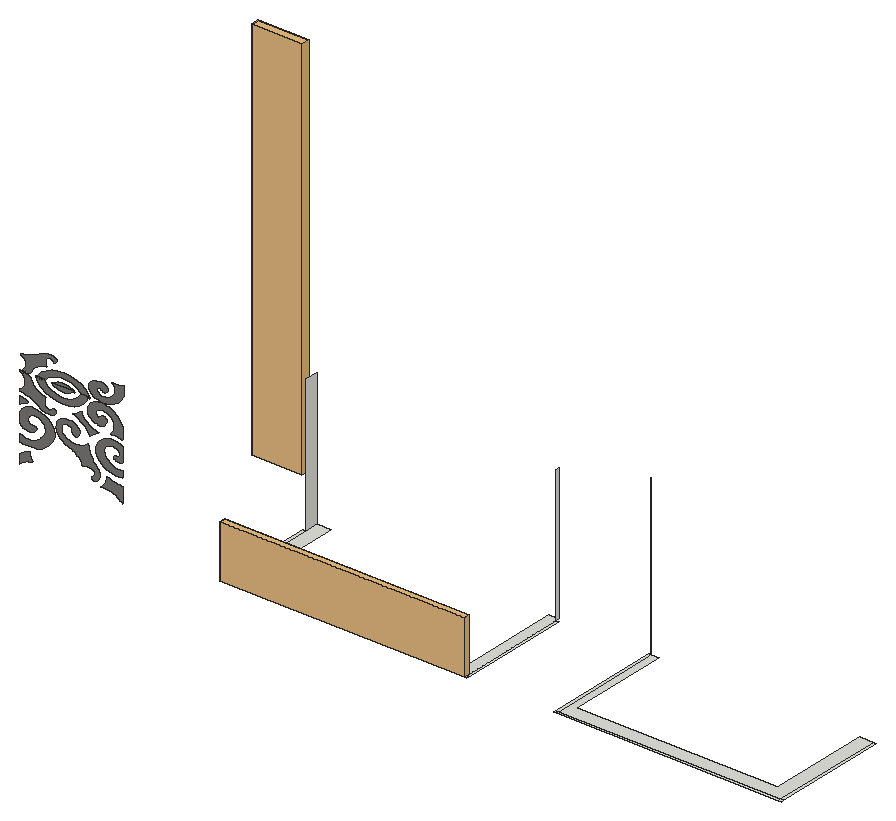
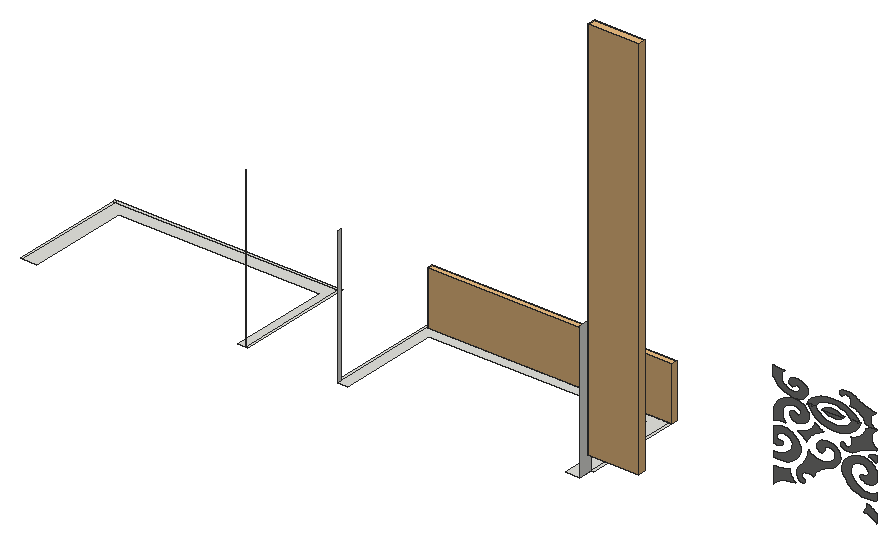
# SketchUp Ruby script. Lengths in inches.
U = 1.inch
M = Sketchup.active_model
def pt(a) = Geom::Point3d.new(a.map { |v| v * U })
def face(e, loops, mat)
  f = e.add_face(loops[0].map { |a| pt(a) })
  loops[1..].each { |l| e.add_face(l.map { |a| pt(a) }).erase! }
  f.material = f.back_material = mat if mat
  f
end
# faces: each face lists its corners as indices into pts; further lists are holes
def faces(e, pts, list, mat = nil) = list.each { |f| face(e, (f[0].is_a?(Array) ? f : [f]).map { |l| l.map { |i| pts[i] } }, mat) }
# xy, xz, yz: faces in a plane at the given z, y or x. An outline is a flat list of corners, or four numbers for a rectangle; further outlines are holes
def ring(l) = l.size == 4 ? [[l[0], l[1]], [l[2], l[1]], [l[2], l[3]], [l[0], l[3]]] : l.each_slice(2).to_a
def flat(e, list, mat, &to3) = list.each { |f| face(e, (f[0].is_a?(Array) ? f : [f]).map { |l| ring(l).map { |u, v| to3.(u, v) } }, mat) }
def xy(e, z, list, mat = nil) = flat(e, list, mat) { |x, y| [x, y, z] }
def xz(e, y, list, mat = nil) = flat(e, list, mat) { |x, z| [x, y, z] }
def yz(e, x, list, mat = nil) = flat(e, list, mat) { |y, z| [x, y, z] }
def lines(e, pts, list) = list.each { |a, b| e.add_line(pt(pts[a]), pt(pts[b])) }
# prism: a flat outline (further loops are holes) pulled along v
def prism(e, loops, v, mat = nil)
  f = face(e, loops, mat); d = Geom::Vector3d.new(v.map { |x| x * U })
  f.pushpull(f.normal.samedirection?(d) ? d.length : -d.length)
end
def box(e, o, s, mat = nil) = prism(e, [[o, [o[0] + s[0], o[1], o[2]], [o[0] + s[0], o[1] + s[1], o[2]], [o[0], o[1] + s[1], o[2]]]], [0, 0, s[2]], mat)
def at(x, y, z, deg = 0) = Geom::Transformation.translation(pt([x, y, z])) * Geom::Transformation.rotation(ORIGIN, Z_AXIS, deg.degrees)
def axes(o, x, y, z) = Geom::Transformation.new([*x, 0, *y, 0, *z, 0, *pt(o).to_a, 1])
def part(name) = M.definitions.add(name)
# library, detail: a bought-in or finely detailed component or shape, given as its bounding box
def library(name, o, s) = part(name).tap { |d| box(d.entities, o, s) }
def detail(e, o, s) = box(e.add_group.entities, o, s)
def put(e, d, t, mat = nil) = e.add_instance(d, t).tap { |i| i.material = mat if mat }
def group(e, t, mat = nil) = e.add_group.tap { |g| g.transformation = t; g.material = mat if mat }.entities
root = M.entities
M.materials.add("[0043_SaddleBrown]4").color = [124, 123, 122]
M.materials.add("[Granite Light Gray]").color = [149, 148, 144]
c1 = library("Scandinavian Door w/ Glass Wall\#2",[-41.94,78.85,0],[6.47,62.99,82.68])
c2 = library("Glass Railing",[0,0,0],[139.5,4.76,42])
xy(root,413.5,[[3051.26,557.9375,3243.69,559.875],[3243.69,557.9375,3245.63,559.875],[3314.21,557.9375,3316.14,559.875],[3316.14,557.9375,3491.44,559.875],[3491.44,557.9375,3493.37,559.875],
  [3051.07,559.875,3053.01,640.11],[3053.01,559.875,3243.69,559.875,3243.69,651.03,3235.84,651.03,3235.84,570.83,3064.33,570.83,3064.33,651.03,3053.01,651.03],[3243.69,559.875,3245.63,647.91],[3314.21,559.875,3316.14,651.03],[3316.14,559.875,3491.44,559.875,3491.44,651.03,3480.11,651.03,3480.11,570.83,3322.22,570.83,3322.22,651.03,3316.14,651.03],
  [3491.44,559.875,3493.37,651.03]])
xz(root,589.17,[[2949.62,418.4,2949.62,430.94,2948.58,430.96,2947.54,431.01,2946.51,431.09,2945.48,431.2,2944.46,431.34,2943.45,431.51,2942.44,431.7,2941.45,431.93,2940.47,432.18,2939.51,432.46,2938.5625,432.77,2937.63,433.11,2937.53,432.33,2937.37,431.56,2937.16,430.79,2936.89,430.03,2936.57,429.29,2936.2,428.55,2935.78,427.83,2935.3,427.13,2934.78,426.44,2934.21,425.78,2933.59,425.14,2932.93,424.52,2934.59,424.625,2936.25,424.61,2937.9,424.48,2939.52,424.22,2941.1,423.85,2942.61,423.36,2944.05,422.76,2945.4,422.0625,2946.64,421.27,2947.77,420.39,2948.76,419.43],[2869.23,418.5,2869.75,419.14,2870.34,419.74,2870.99,420.3125,2871.71,420.84,2872.49,421.32,2873.32,421.76,2874.19,422.14,2875.11,422.48,2876.06,422.75,2877.03,422.98,2878.03,423.14,2879.05,423.24,2878.63,423.73,2878.25,424.24,2877.9,424.76,2877.6,425.29,2877.33,425.83,2877.1,426.38,2876.91,426.94,2876.76,427.51,2876.65,428.08,2876.58,428.65,2876.55,429.23,2876.57,429.8,2875.87,429.54,2875.19,429.27,2874.51,428.97,2873.86,428.66,2873.22,428.33,2872.59,427.99,2871.98,427.63,2871.39,427.26,2870.82,426.87,2870.27,426.47,2869.74,426.05,2869.23,425.62],[2927.3,427.2,2927.86,427.23,2928.4,427.32,2928.93,427.46,2929.41,427.66,2929.86,427.9,2930.25,428.18,2930.58,428.51,2930.85,428.86,2931.04,429.24,2931.16,429.63,2931.19,430.04,2931.41,430.71,2931.55,431.38,2931.63,432.07,2931.64,432.76,2931.57,433.44,2931.44,434.125,2931.24,434.8,2930.98,435.46,2930.64,436.1,2930.24,436.72,2929.79,437.33,2929.27,437.9,2928.33,438.91,2927.46,439.95,2926.66,441.02,2925.92,442.11,2925.25,443.22,2924.66,444.36,2924.13,445.51,2923.68,446.68,2923.3,447.86,2923,449.05,2922.77,450.26,2922.62,451.46,2921.65,450.57,2920.53,449.77,2919.28,449.08,2917.91,448.52,2916.45,448.09,2914.93,447.8,2913.37,447.66,2911.79,447.66,2910.23,447.8125,2908.71,448.11,2907.26,448.54,2905.89,449.11,2904.92,449.65,2904.05,450.27,2903.3,450.97,2902.68,451.74,2902.2,452.55,2901.875,453.4,2901.7,454.28,2901.68,455.16,2901.82,456.04,2902.12,456.9,2902.57,457.72,2903.16,458.5,2903.7,458.79,2904.31,459.03,2904.95,459.19,2905.62,459.29,2906.3,459.31,2906.98,459.26,2907.64,459.13,2908.27,458.94,2908.85,458.68,2909.37,458.36,2909.82,457.99,2910.1875,457.57,2910.07,457.28,2909.98,456.98,2909.93,456.67,2909.91,456.37,2909.92,456.06,2909.97,455.75,2910.05,455.45,2910.16,455.16,2910.31,454.87,2910.49,454.59,2910.7,454.32,2910.93,454.0625,2911.16,453.87,2911.4375,453.7,2911.74,453.5625,2912.07,453.47,2912.42,453.41,2912.78,453.38,2913.14,453.41,2913.48,453.47,2913.82,453.5625,2914.12,453.7,2914.39,453.87,2914.625,454.0625,2915.3,454.87,2915.77,455.75,2916.03,456.67,2916.0625,457.61,2915.875,458.54,2915.47,459.4375,2914.85,460.27,2914.05,461.01,2913.09,461.64,2911.99,462.15,2910.78,462.51,2909.51,462.72,2908.09,462.91,2906.65,462.94,2905.21,462.8125,2903.83,462.53,2902.51,462.1,2901.3,461.53,2900.23,460.83,2899.32,460.03,2898.58,459.13,2898.04,458.17,2897.72,457.15,2897.61,456.12,2897.49,454.92,2897.56,453.72,2897.79,452.53,2898.19,451.37,2898.76,450.24,2899.49,449.16,2900.37,448.14,2901.39,447.19,2902.54,446.32,2903.81,445.55,2905.18,444.87,2906.65,444.3,2908.04,443.78,2909.37,443.1875,2910.64,442.53,2911.85,441.81,2912.98,441.03,2914.03,440.19,2914.99,439.31,2915.87,438.37,2916.65,437.39,2917.34,436.38,2917.92,435.33,2918.4,434.26,2919.08,434.625,2919.82,434.93,2920.61,435.15,2921.43,435.3,2922.28,435.36,2923.13,435.34,2923.97,435.24,2924.78,435.05,2925.55,434.79,2926.26,434.46,2926.9,434.06,2927.47,433.6,2927.67,433.23,2927.82,432.84,2927.9,432.45,2927.93,432.05,2927.89,431.65,2927.78,431.26,2927.62,430.875,2927.4,430.51,2927.125,430.16,2926.79,429.84,2926.42,429.55,2926,429.29,2925.77,429.13,2925.58,428.95,2925.45,428.75,2925.38,428.53,2925.37,428.3,2925.42,428.08,2925.53,427.87,2925.69,427.67,2925.9,427.51,2926.16,427.375,2926.44,427.28,2926.75,427.23],[2875.84,433.3,2878.1,433.36,2880.34,433.62,2882.51,434.07,2884.6,434.7,2886.5625,435.5,2888.38,436.47,2890.02,437.59,2891.47,438.85,2892.7,440.22,2894.37,442.26,2895.52,444.47,2896.14,446.8,2896.18,449.17,2895.66,451.51,2894.59,453.75,2893,455.82,2890.9375,457.67,2888.46,459.23,2885.66,460.46,2882.6,461.32,2879.38,461.79,2878.22,461.63,2877.08,461.4,2875.99,461.08,2874.9375,460.69,2873.94,460.24,2873.01,459.71,2872.16,459.125,2871.38,458.48,2870.7,457.79,2870.11,457.06,2869.61,456.28,2869.23,455.48,2869.23,447.4,2869.76,446.49,2870.53,445.68,2871.52,445,2872.68,444.48,2873.96,444.15,2875.3,444,2876.67,444.0625,2877.98,444.32,2879.2,444.76,2880.26,445.37,2881.13,446.13,2881.77,447,2881.87,447.21,2881.92,447.42,2881.92,447.64,2881.88,447.86,2881.8,448.07,2881.67,448.27,2881.51,448.46,2881.31,448.62,2881.07,448.76,2880.82,448.88,2880.54,448.97,2880.24,449.02,2879.51,448.93,2878.78,448.94,2878.06,449.05,2877.375,449.25,2876.75,449.54,2876.22,449.9,2875.78,450.33,2875.47,450.81,2875.28,451.32,2875.22,451.85,2875.31,452.38,2875.52,452.89,2875.7,453.55,2876.03,454.18,2876.49,454.77,2877.07,455.29,2877.76,455.75,2878.53,456.12,2879.38,456.4,2880.28,456.57,2881.21,456.65,2882.14,456.62,2883.06,456.48,2883.93,456.24,2885.28,455.45,2886.47,454.53,2887.47,453.51,2888.25,452.39,2888.8125,451.2,2889.13,449.96,2889.2,448.71,2889.03,447.46,2888.61,446.24,2887.96,445.08,2887.09,443.99,2886.01,443.01,2885.57,442.35,2885.06,441.73,2884.47,441.14,2883.83,440.59,2883.12,440.07,2882.35,439.6,2881.53,439.18,2880.67,438.8125,2879.76,438.49,2878.82,438.23,2877.86,438.03,2876.875,437.88,2876.17,437.82,2875.47,437.8,2874.76,437.83,2874.0625,437.89,2873.37,438,2872.7,438.16,2872.04,438.35,2871.41,438.58,2870.8125,438.85,2870.24,439.15,2869.71,439.48,2869.23,439.85,2869.23,434.28,2871.37,433.76,2873.59,433.44],[2947.02,436.71,2949.62,436.96,2949.62,441.66,2947.39,441.61,2945.18,441.84,2943.06,442.34,2941.09,443.09,2939.33,444.09,2937.84,445.28,2936.66,446.65,2935.83,448.14,2935.37,449.72,2935.3,451.32,2935.62,452.92,2936.3125,454.45,2937.11,455.1,2938.06,455.63,2939.13,456.03,2940.29,456.27,2941.49,456.35,2942.7,456.27,2943.85,456.02,2944.93,455.625,2945.875,455.09,2946.67,454.43,2947.28,453.68,2947.68,452.86,2947.75,452.53,2947.74,452.1875,2947.66,451.86,2947.49,451.54,2947.25,451.25,2946.95,450.99,2946.59,450.77,2946.1875,450.61,2945.75,450.49,2945.29,450.43,2944.82,450.42,2944.36,450.48,2944.12,450.4,2943.89,450.31,2943.68,450.19,2943.48,450.06,2943.31,449.92,2943.15,449.77,2943.03,449.6,2942.92,449.42,2942.85,449.24,2942.8,449.06,2942.78,448.87,2942.79,448.68,2943.15,448.29,2943.59,447.9375,2944.09,447.63,2944.64,447.38,2945.23,447.18,2945.85,447.04,2946.49,446.96,2947.14,446.9375,2947.79,446.98,2948.43,447.09,2949.04,447.25,2949.62,447.47,2949.62,459.11,2948.55,459.72,2947.4,460.23,2946.16,460.64,2944.87,460.9375,2943.53,461.12,2942.18,461.18,2940.82,461.12,2939.48,460.9375,2938.1875,460.64,2936.95,460.23,2935.8,459.72,2934.74,459.11,2933.84,458.48,2933.01,457.82,2932.24,457.11,2931.53,456.375,2930.9,455.6,2930.34,454.8,2929.86,453.97,2929.45,453.125,2929.125,452.26,2928.88,451.38,2928.72,450.49,2928.64,449.6,2928.75,447.71,2929.26,445.86,2930.15,444.08,2931.4,442.42,2932.98,440.92,2934.86,439.6,2936.99,438.5,2939.33,437.65,2941.82,437.06,2944.4,436.74],
  [2923.72,457.23,2924.27,457.6875,2924.83,458.14,2925.41,458.59,2925.99,459.03,2926.58,459.46,2927.18,459.89,2927.79,460.31,2928.41,460.72,2929.04,461.12,2929.68,461.52,2930.32,461.91,2930.98,462.29,2929.32,462.61,2927.71,463.04,2926.17,463.58,2924.7,464.23,2923.34,464.99,2922.08,465.83,2920.95,466.76,2919.94,467.77,2919.08,468.84,2918.37,469.96,2917.81,471.14,2917.42,472.34,2916.94,471.93,2916.4375,471.54,2915.91,471.16,2915.37,470.79,2914.8125,470.43,2914.23,470.09,2913.64,469.77,2913.03,469.47,2912.4,469.18,2911.76,468.9,2911.1,468.65,2910.4375,468.41,2912,467.83,2913.5,467.18,2914.9375,466.45,2916.3,465.65,2917.57,464.79,2918.76,463.86,2919.85,462.87,2920.85,461.83,2921.73,460.74,2922.51,459.6,2923.18,458.43],[2869.23,460.92,2869.64,461.25,2870.08,461.57,2870.53,461.88,2871.01,462.17,2871.5,462.45,2872.01,462.71,2872.53,462.95,2873.07,463.18,2873.62,463.39,2874.18,463.58,2874.76,463.75,2875.34,463.91,2874.96,464.24,2874.55,464.55,2874.11,464.84,2873.64,465.11,2873.15,465.35,2872.63,465.56,2872.1,465.76,2871.55,465.92,2870.98,466.05,2870.4,466.16,2869.82,466.24,2869.23,466.28],[2891.28,461.65,2892.2,461.6875,2893.11,461.8,2894,461.98,2894.85,462.23,2895.16,462.34,2895.45,462.47,2895.72,462.62,2895.98,462.79,2896.21,462.96,2896.43,463.16,2896.62,463.36,2896.79,463.58,2896.93,463.8,2897.04,464.03,2897.13,464.27,2897.19,464.52,2897.22,464.75,2897.2,464.99,2897.15,465.23,2897.07,465.46,2896.94,465.6875,2896.79,465.9,2896.59,466.1,2896.375,466.28,2896.125,466.4375,2895.85,466.58,2895.5625,466.69,2895.25,466.78,2895.0625,466.54,2894.86,466.29,2894.64,466.06,2894.18,465.6,2893.93,465.38,2893.67,465.17,2893.4,464.96,2893.12,464.77,2892.83,464.57,2892.53,464.39,2892.22,464.21,2891.8,464.28,2891.39,464.375,2890.99,464.5,2890.61,464.65,2890.25,464.83,2889.92,465.03,2889.61,465.26,2889.34,465.5,2889.11,465.77,2888.91,466.04,2888.74,466.33,2888.62,466.63,2888.48,467.11,2888.37,467.58,2888.29,468.0625,2888.25,468.55,2888.24,469.03,2888.26,469.51,2888.3125,469.99,2888.4,470.47,2888.52,470.95,2888.67,471.42,2888.85,471.88,2889.07,472.34,2887.6,472.75,2886.1875,473.24,2884.84,473.83,2883.57,474.5,2882.39,475.24,2881.31,476.0625,2880.33,476.95,2879.46,477.9,2878.72,478.89,2878.1,479.94,2877.61,481.01,2877.26,482.12,2876.88,482.3,2876.51,482.48,2876.14,482.68,2875.79,482.88,2875.4375,483.09,2875.1,483.31,2874.77,483.53,2874.45,483.77,2874.14,484.01,2873.84,484.25,2873.55,484.5,2873.27,484.8,2869.23,484.8,2869.23,483.92,2870.3125,483.03,2871.23,482.05,2871.96,480.99,2872.49,479.87,2872.8125,478.71,2872.92,477.53,2872.8125,476.35,2872.49,475.1875,2871.96,474.07,2871.23,473.01,2870.3125,472.02,2869.23,471.14,2869.23,469.95,2870.7,469.73,2872.15,469.45,2873.58,469.11,2874.99,468.72,2876.36,468.27,2877.69,467.77,2878.98,467.21,2880.23,466.61,2881.4375,465.96,2882.59,465.26,2883.68,464.51,2884.72,463.73,2885.37,463.26,2886.09,462.84,2886.86,462.48,2887.6875,462.18,2888.55,461.94,2889.44,461.77,2890.36,461.68],[2949.62,463.51,2949.62,472.52,2949.2,473.85,2948.61,475.15,2947.85,476.4,2946.92,477.6,2945.84,478.72,2944.61,479.76,2943.25,480.71,2941.77,481.57,2940.19,482.3125,2938.51,482.95,2936.75,483.46,2934.93,483.85,2933.26,483.91,2931.6,483.79,2929.99,483.49,2928.45,483.03,2927.02,482.4,2925.74,481.63,2924.63,480.73,2923.72,479.72,2923.03,478.625,2922.57,477.47,2922.35,476.28,2922.38,475.07,2922.33,474.3125,2922.41,473.55,2922.62,472.81,2922.95,472.09,2923.4,471.4,2923.97,470.76,2924.64,470.17,2925.4,469.64,2926.25,469.1875,2927.16,468.81,2928.14,468.51,2929.15,468.31,2929.83,468.02,2930.56,467.82,2931.34,467.71,2932.125,467.7,2932.9,467.78,2933.65,467.96,2934.34,468.22,2934.96,468.57,2935.49,468.99,2935.92,469.47,2936.22,469.99,2936.4,470.54,2936.8,470.95,2937.09,471.4,2937.28,471.88,2937.34,472.38,2937.29,472.88,2937.12,473.36,2936.83,473.81,2936.45,474.23,2935.97,474.59,2935.41,474.88,2934.78,475.1,2934.12,475.24,2933.89,474.99,2933.64,474.75,2933.39,474.52,2933.125,474.29,2932.85,474.07,2932.5625,473.85,2932.27,473.64,2931.96,473.44,2931.65,473.25,2931.32,473.0625,2930.99,472.88,2930.65,472.71,2930.28,472.88,2929.94,473.08,2929.62,473.31,2929.34,473.55,2929.1,473.82,2928.91,474.1,2928.75,474.4,2928.64,474.71,2928.58,475.02,2928.57,475.34,2928.6,475.66,2928.68,475.97,2928.97,476.6,2929.39,477.18,2929.9375,477.71,2930.6,478.17,2931.35,478.54,2932.18,478.83,2933.06,479.01,2933.97,479.09,2934.88,479.06,2935.78,478.93,2936.64,478.7,2937.43,478.36,2938.85,477.55,2940.1,476.6,2941.16,475.54,2942.01,474.39,2942.64,473.16,2943.03,471.88,2943.18,470.58,2943.09,469.28,2942.75,467.99,2942.18,466.75,2941.37,465.58,2940.36,464.5,2941.14,464.63,2941.93,464.73,2942.73,464.78,2943.53,464.8,2944.33,464.77,2945.13,464.71,2945.92,464.6,2946.7,464.46,2947.46,464.28,2948.2,464.06,2948.92,463.8],[2902.46,472.34,2907.28,472.75,2911.84,473.95,2915.9,475.88,2919.23,478.43,2921.66,481.46,2923.0625,484.8,2916.91,484.8,2915.73,482.62,2913.92,480.66,2911.57,479.03,2908.78,477.8,2905.7,477.04,2902.45,476.77,2899.21,477.02,2896.11,477.76,2893.3125,478.97,2890.94,480.59,2889.11,482.53,2887.9,484.8,2881.74,484.8,2883.18,481.37,2885.63,478.35,2888.99,475.82,2893.0625,473.91,2897.63,472.73],
  [2902.77,480.9,2904.54,481.02,2906.24,481.375,2907.8125,481.95,2909.21,482.74,2910.375,483.7,2911.27,484.8,2894.28,484.8,2895.17,483.7,2896.34,482.74,2897.73,481.95,2899.3125,481.375,2901.01,481.02],[2869.93,483.9,2869.93,484.65,2871.02,485.41,2871.9375,486.24,2872.67,487.15,2873.2,488.1,2873.52,489.09,2873.625,490.1,2873.52,491.1,2873.2,492.09,2872.67,493.05,2871.9375,493.95,2871.02,494.79,2869.93,495.54,2869.93,496.56,2871.41,496.75,2872.86,496.98,2874.29,497.27,2875.69,497.61,2877.0625,497.99,2878.4,498.41,2879.69,498.89,2880.94,499.4,2882.14,499.96,2883.29,500.55,2884.39,501.1875,2885.43,501.86,2886.08,502.26,2886.8,502.61,2887.57,502.92,2888.39,503.18,2889.26,503.375,2890.15,503.52,2891.0625,503.6,2891.98,503.63,2892.91,503.59,2893.81,503.5,2894.7,503.34,2895.56,503.13,2895.86,503.04,2896.15,502.92,2896.43,502.8,2896.68,502.66,2896.92,502.51,2897.13,502.34,2897.33,502.17,2897.49,501.98,2897.64,501.79,2897.75,501.59,2897.84,501.39,2897.9,501.18,2897.92,500.98,2897.91,500.78,2897.86,500.57,2897.77,500.375,2897.65,500.1875,2897.49,500.01,2897.3,499.84,2897.08,499.68,2896.83,499.55,2896.5625,499.43,2896.27,499.33,2895.96,499.25,2895.77,499.46,2895.56,499.67,2895.35,499.87,2895.12,500.07,2894.88,500.26,2894.63,500.44,2894.375,500.625,2894.1,500.8,2893.83,500.97,2893.54,501.13,2893.24,501.29,2892.93,501.44,2892.51,501.38,2892.09,501.3,2891.69,501.2,2891.31,501.07,2890.96,500.91,2890.625,500.74,2890.32,500.55,2890.05,500.34,2889.8125,500.12,2889.61,499.88,2889.45,499.64,2889.33,499.38,2889.19,498.98,2889.08,498.57,2889,498.16,2888.95,497.75,2888.94,497.34,2888.96,496.93,2889.02,496.52,2889.11,496.11,2889.22,495.7,2889.375,495.3,2889.56,494.91,2889.77,494.52,2888.31,494.17,2886.89,493.75,2885.55,493.25,2884.28,492.68,2883.1,492.05,2882.01,491.35,2881.03,490.59,2880.17,489.78,2879.43,488.93,2878.81,488.05,2878.32,487.13,2877.97,486.1875,2877.59,486.04,2877.21,485.88,2876.49,485.54,2876.14,485.36,2875.48,484.98,2875.16,484.78,2874.85,484.58,2874.55,484.37,2874.26,484.16,2873.98,483.9],[2882.45,483.9,2883.88,486.82,2886.34,489.4,2889.7,491.55,2893.77,493.18,2898.34,494.1875,2903.17,494.52,2907.99,494.17,2912.55,493.14,2916.6,491.5,2919.9375,489.33,2922.37,486.75,2923.77,483.9,2917.61,483.9,2916.43,485.76,2914.625,487.43,2912.27,488.82,2909.49,489.86,2906.4,490.51,2903.16,490.74,2899.92,490.53,2896.82,489.9,2894.02,488.87,2891.65,487.49,2889.82,485.83,2888.61,483.9],[2894.98,483.9,2895.88,484.84,2897.05,485.66,2898.44,486.33,2900.02,486.82,2901.72,487.125,2903.48,487.23,2905.24,487.125,2906.94,486.82,2908.52,486.33,2909.92,485.66,2911.08,484.84,2911.98,483.9],[2933.97,484.66,2932.3125,484.76,2930.69,485.02,2929.15,485.41,2927.73,485.95,2926.45,486.6,2925.34,487.37,2924.43,488.23,2923.73,489.16,2923.27,490.15,2923.05,491.16,2923.08,492.1875,2923.04,492.84,2923.12,493.48,2923.33,494.12,2923.66,494.73,2924.11,495.32,2924.68,495.87,2925.34,496.37,2926.11,496.82,2926.95,497.21,2927.87,497.53,2928.84,497.78,2929.86,497.95,2930.54,498.2,2931.27,498.37,2932.04,498.46,2932.83,498.48,2933.61,498.4,2934.36,498.25,2935.05,498.02,2935.67,497.73,2936.2,497.37,2936.625,496.96,2936.93,496.52,2937.11,496.05,2937.5,495.7,2937.8,495.32,2937.98,494.91,2938.05,494.48,2938,494.0625,2937.83,493.65,2937.54,493.26,2937.15,492.91,2936.67,492.6,2936.11,492.35,2935.49,492.17,2934.83,492.05,2934.59,492.26,2934.35,492.46,2934.1,492.66,2933.83,492.86,2933.55,493.05,2933.27,493.23,2932.97,493.41,2932.67,493.58,2932.03,493.9,2931.7,494.05,2931.36,494.2,2930.99,494.05,2930.64,493.89,2930.33,493.7,2930.05,493.49,2929.8125,493.26,2929.61,493.02,2929.46,492.76,2929.35,492.5,2929.29,492.23,2929.27,491.96,2929.31,491.69,2929.39,491.43,2929.67,490.89,2930.1,490.39,2930.65,489.94,2931.31,489.55,2932.06,489.23,2932.89,488.99,2933.77,488.83,2934.68,488.77,2935.59,488.79,2936.49,488.9,2937.34,489.1,2938.14,489.39,2939.55,490.08,2940.8,490.89,2941.86,491.79,2942.72,492.77,2943.35,493.82,2943.74,494.91,2943.89,496.02,2943.8,497.13,2943.46,498.22,2942.88,499.28,2942.08,500.28,2941.06,501.2,2941.85,501.09,2942.64,501.01,2943.4375,500.96,2944.24,500.95,2945.04,500.97,2945.84,501.02,2946.63,501.11,2947.41,501.23,2948.17,501.39,2948.91,501.57,2949.63,501.79,2950.32,502.04,2950.32,494.37,2949.91,493.23,2949.32,492.125,2948.55,491.06,2947.63,490.04,2946.55,489.08,2945.32,488.2,2943.96,487.38,2942.48,486.66,2940.89,486.02,2939.21,485.48,2937.46,485.04,2935.64,484.71]],"[0043_SaddleBrown]4")
xz(root,651.03,[[3315.93,413.5,3316.14,538.1875]])
yz(root,3053.01,[[640.11,413.5,651.03,520.4375]])
yz(root,3243.69,[[647.91,413.5,651.03,520.4375]])
p = [[2869.23,589.17,469.95],[2869.23,589.17,466.28]]
lines(root,p,[[0,1]])
put(root,c1,axes([2947.5,621.1,440.32],[0,-1,0],[0.63229,0,0],[0,0,3.672]))
put(root,c2,axes([3051.26,557.9375,413.5],[1.37946,0,0],[0,1,0],[0,0,1]),"[Granite Light Gray]")
